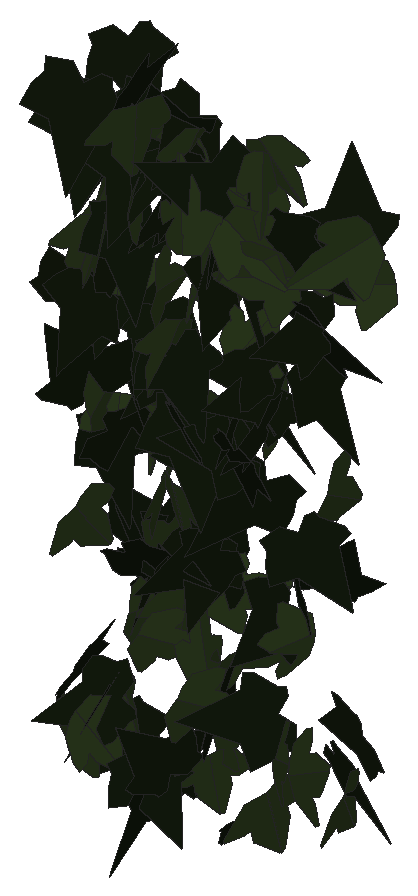
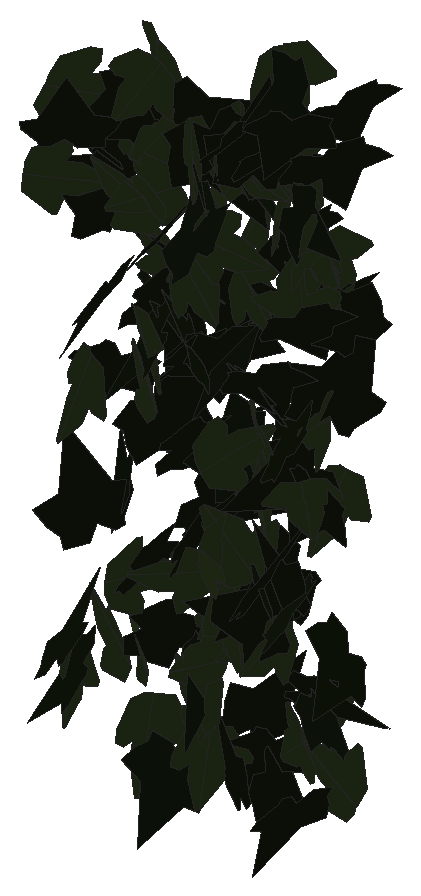
# SketchUp Ruby script. Lengths in inches.
U = 1.inch
M = Sketchup.active_model
def pt(a) = Geom::Point3d.new(a.map { |v| v * U })
def face(e, loops, mat)
  f = e.add_face(loops[0].map { |a| pt(a) })
  loops[1..].each { |l| e.add_face(l.map { |a| pt(a) }).erase! }
  f.material = f.back_material = mat if mat
  f
end
# faces: each face lists its corners as indices into pts; further lists are holes
def faces(e, pts, list, mat = nil) = list.each { |f| face(e, (f[0].is_a?(Array) ? f : [f]).map { |l| l.map { |i| pts[i] } }, mat) }
# xy, xz, yz: faces in a plane at the given z, y or x. An outline is a flat list of corners, or four numbers for a rectangle; further outlines are holes
def ring(l) = l.size == 4 ? [[l[0], l[1]], [l[2], l[1]], [l[2], l[3]], [l[0], l[3]]] : l.each_slice(2).to_a
def flat(e, list, mat, &to3) = list.each { |f| face(e, (f[0].is_a?(Array) ? f : [f]).map { |l| ring(l).map { |u, v| to3.(u, v) } }, mat) }
def xy(e, z, list, mat = nil) = flat(e, list, mat) { |x, y| [x, y, z] }
def xz(e, y, list, mat = nil) = flat(e, list, mat) { |x, z| [x, y, z] }
def yz(e, x, list, mat = nil) = flat(e, list, mat) { |y, z| [x, y, z] }
def lines(e, pts, list) = list.each { |a, b| e.add_line(pt(pts[a]), pt(pts[b])) }
# prism: a flat outline (further loops are holes) pulled along v
def prism(e, loops, v, mat = nil)
  f = face(e, loops, mat); d = Geom::Vector3d.new(v.map { |x| x * U })
  f.pushpull(f.normal.samedirection?(d) ? d.length : -d.length)
end
def box(e, o, s, mat = nil) = prism(e, [[o, [o[0] + s[0], o[1], o[2]], [o[0] + s[0], o[1] + s[1], o[2]], [o[0], o[1] + s[1], o[2]]]], [0, 0, s[2]], mat)
def at(x, y, z, deg = 0) = Geom::Transformation.translation(pt([x, y, z])) * Geom::Transformation.rotation(ORIGIN, Z_AXIS, deg.degrees)
def axes(o, x, y, z) = Geom::Transformation.new([*x, 0, *y, 0, *z, 0, *pt(o).to_a, 1])
def part(name) = M.definitions.add(name)
# library, detail: a bought-in or finely detailed component or shape, given as its bounding box
def library(name, o, s) = part(name).tap { |d| box(d.entities, o, s) }
def detail(e, o, s) = box(e.add_group.entities, o, s)
def put(e, d, t, mat = nil) = e.add_instance(d, t).tap { |i| i.material = mat if mat }
def group(e, t, mat = nil) = e.add_group.tap { |g| g.transformation = t; g.material = mat if mat }.entities
root = M.entities
M.materials.add("efeu1").color = [18, 25, 13]
M.materials.add("efeu2").color = [43, 57, 29]
c1 = part("ivyleaf_10")
p = [[0,0.5,-0.03],[-0.0625,2.02,-0.43],[-0.19,2.01,-0.46],[-0.54,1.05,-0.29],[-0.52,0.625,-0.18],[-0.83,0.76,-0.28],
  [-1.16,0.64,-0.33],[-1.15,0.33,-0.24],[-0.77,-0.39,0.02],[-0.3,-0.51,0.16],[0.04,-0.48,0.23],[-0.02,2.01,-0.4375],
  [-0.06,2.01,-0.43],[0.04,-0.49,0.23],[0.67,-0.49,0.14],[1.38,0.36,-0.2],[1.375,0.51,-0.24],[0.81,0.65,-0.19],
  [0.62,0.59,-0.15],[0.6,1.09,-0.28],[0.5,1.23,-0.31]]
faces(c1.entities,p,[[0,1,2,3,4,5,6,7,8,9,10],[11,12,0,13,14,15,16,17,18,19,20]],"efeu2")
c2 = part("ivyleaf_9")
p = [[1.54,2.16,1.25],[1.36,2.04,1.19],[-0.21,0.99,0.68],[-0.71,1.11,0.82],[-0.85,0.86,0.67],[-0.8,0.17,0.21],
  [-0.9,-0.01,0.1],[-0.67,-0.16,-0.02],[-0.08,-0.08,-0.05],[-0.03,-0.6,-0.4],[0.65,-0.88,-0.66],[0.83,-0.6,-0.49],
  [1.29,-0.42,-0.43],[1.8125,-0.07,-0.26],[1.21,0.44,0.15]]
faces(c2.entities,p,[[0,1,2,3,4,5,6,7,8,9,10,11,12,13,14]],"efeu1")
put(root,c1,axes([551.7,129.9,193.51],[-0.22343,-0.76212,-0.59809],[0.1909,0.56712,-0.79397],[0.94979,-0.29327,0.01889]))
put(root,c2,axes([557.02,130.01,197.18],[0.67195,0.09743,-0.58653],[-0.58638,-0.03779,-0.67805],[-0.09833,0.89112,0.03537]))
put(root,c2,axes([551.27,130.98,199.67],[-0.22153,-0.82284,0.36012],[-0.09205,-0.34816,-0.85214],[0.89346,-0.23989,0.0015]))
put(root,c1,axes([553.25,130.34,206.24],[-0.39364,-0.98437,-0.06429],[0.02505,0.05922,-1.06016],[0.98615,-0.39443,0.00127]))
put(root,c2,axes([550.91,130.95,206.06],[-0.26139,-1.01728,-0.03229],[0.00866,0.03112,-1.05033],[1.01776,-0.26153,0.00064]))
put(root,c1,axes([551.83,130,186.88],[0.07493,0.79738,0.51971],[0.03298,0.51883,-0.80078],[-0.95122,0.0808,0.01317]))
put(root,c2,axes([553.98,130.88,185.74],[0.22147,0.16104,0.80389],[-0.69624,-0.40278,0.27249],[0.43293,-0.73011,0.02699]))
put(root,c2,axes([559.02,130.34,195.12],[-0.08835,-0.46455,-0.74307],[0.27342,0.69494,-0.46697],[0.83258,-0.27751,0.0745]))
put(root,c2,axes([557.65,130.48,197.96],[-0.64583,0.58215,-0.09351],[0.06994,-0.06207,-0.86948],[-0.58545,-0.64961,-0.00072]))
put(root,c2,axes([554.7,130.26,197.55],[0.90407,-0.29541,-0.45534],[-0.41902,0.18244,-0.95031],[0.34501,0.99569,0.03903]))
put(root,c1,axes([554.12,130.89,199.51],[-0.01362,-0.86994,0.34595],[0.05119,-0.34616,-0.86845],[0.9348,0.00628,0.0526]))
put(root,c2,axes([555.11,130.9,197.27],[-0.42388,-0.91668,-0.39818],[0.17401,0.35821,-1.00992],[0.98416,-0.45816,0.00707]))
put(root,c2,axes([552.19,130.91,187.42],[-0.74149,-0.04215,0.44705],[-0.44726,-0.00721,-0.74252],[0.03982,-0.8658,-0.01558]))
put(root,c1,axes([554.85,130.5,203.06],[1.00737,-0.17015,0.32042],[-0.31494,0.05924,1.02162],[-0.18007,-1.05544,0.00569]))
put(root,c1,axes([556.63,130.51,203.66],[0.54869,0.18477,0.81134],[0.74743,0.3177,-0.57783],[-0.36572,0.9265,0.03634]))
put(root,c2,axes([559.39,130.69,201.47],[-0.77674,0.32028,0.27419],[-0.25521,0.10031,-0.84017],[-0.3356,-0.81758,0.00433]))
put(root,c2,axes([554.34,130.76,199.15],[-0.34514,-0.49854,-0.67397],[0.48534,0.47546,-0.60023],[0.68353,-0.58932,0.08589]))
put(root,c2,axes([556.11,131.41,196.45],[0.02498,-0.78714,-0.50493],[0.01742,-0.50463,0.78754],[-0.93501,-0.03043,0.00118]))
put(root,c1,axes([557.09,130.94,205.66],[0.78124,-0.3259,0.37248],[0.35968,-0.10427,-0.84561],[0.33998,0.85919,0.03867]))
put(root,c2,axes([551.44,129.99,188.44],[0.08878,0.71867,0.61151],[0.06846,0.60768,-0.72412],[-0.94114,0.112,0.00501]))
put(root,c1,axes([557.88,130.78,202.625],[0.30428,0.05979,-0.98206],[-0.98175,0.08596,-0.29895],[0.06462,1.02451,0.08239]))
put(root,c1,axes([551.5,130.85,201.88],[0.72615,-0.72293,-0.12259],[-0.07186,0.10154,-1.02444],[0.72972,0.72939,0.02111]))
put(root,c2,axes([551.02,131.18,196.66],[0.50959,0.22223,0.84296],[-0.76823,-0.34706,0.55591],[0.41207,-0.92185,-0.00607]))
put(root,c2,axes([553.09,131.34,184.76],[-0.31411,0.29431,-0.81585],[0.5311,-0.62073,-0.4284],[-0.68569,-0.61561,0.04192]))
put(root,c1,axes([554.15,130.29,201.26],[0.06734,-0.27016,-0.88247],[-0.02663,0.88387,-0.27262],[0.92251,0.04524,0.05654]))
put(root,c2,axes([551.68,131.1,187.39],[-0.52529,0.5187,-0.44741],[0.29735,-0.33527,-0.73779],[-0.6171,-0.60308,0.02535]))
put(root,c2,axes([555.11,131.58,192.72],[-0.15654,-0.10174,-0.85456],[0.0375,-0.86856,0.09653],[-0.85977,-0.01936,0.1598]))
put(root,c1,axes([551.05,131.25,201.6],[-0.20787,-0.89241,0.2302],[0.00276,-0.23659,-0.91467],[0.92162,-0.20057,0.05466]))
put(root,c2,axes([553.11,131,185.56],[-0.21555,-0.50578,-0.64108],[0.25947,0.58625,-0.54976],[0.77425,-0.33728,0.00577]))
put(root,c2,axes([555.98,131.38,203.95],[-0.32139,0.10096,1.00271],[-1.00772,-0.04337,-0.31863],[0.0107,-1.05206,0.10936]))
put(root,c2,axes([557.25,131.05,199.4],[-0.64746,0.34529,0.47022],[-0.43417,0.18399,-0.73293],[-0.38965,-0.77876,0.03533]))
put(root,c1,axes([558.09,131.5,186.86],[0.3952,-0.30601,-0.93342],[0.70563,-0.61151,0.49924],[-0.68338,-0.80839,-0.02431]))
put(root,c2,axes([555.79,130.87,196.5],[-0.30539,0.7564,0.28371],[0.02381,-0.29475,0.81146],[0.80751,0.29476,0.08337]))
put(root,c1,axes([557.22,131.63,187.02],[0.17803,-0.28673,-0.85954],[0.48288,-0.71119,0.33726],[-0.76671,-0.51449,0.01282]))
put(root,c2,axes([557,131.87,198.33],[0.11039,-0.57035,-0.66871],[0.12538,-0.65685,0.58094],[-0.86992,-0.16705,-0.00113]))
put(root,c1,axes([554.93,130.61,188.43],[-0.29325,-0.4429,-0.82357],[0.44216,0.69486,-0.53112],[0.82397,-0.53051,-0.0081]))
put(root,c2,axes([550.4,131,199.26],[-0.19451,-0.02702,0.88712],[0.87275,-0.17085,0.18616],[0.16127,0.89198,0.06253]))
put(root,c1,axes([559.89,131.74,203.9],[0.30916,0.3457,-0.98261],[-0.66001,-0.72796,-0.46376],[-0.80587,0.72882,0.00286]))
put(root,c1,axes([554.79,131.32,201.75],[0.59137,-0.71726,0.00658],[0.00422,-0.00505,-0.92962],[0.71728,0.59139,0.00004]))
put(root,c1,axes([554.2,131.01,194.48],[-0.77999,0.3281,0.11887],[-0.11176,0.04089,-0.84617],[-0.33059,-0.78794,0.00559]))
put(root,c2,axes([552.04,131.5,202.01],[-0.02236,-0.96485,-0.17622],[0.01726,0.17585,-0.96502],[0.98066,-0.0251,0.01297]))
put(root,c2,axes([558.46,131.46,200.82],[0.52594,-0.45764,0.81289],[0.65675,-0.48107,-0.69575],[0.66249,0.84022,0.04439]))
put(root,c2,axes([557.6,130.98,203.78],[0.011,-0.07092,-0.97432],[0.64691,0.73065,-0.04588],[0.73201,-0.64465,0.05518]))
put(root,c2,axes([552.42,131.75,204.1],[-0.56426,-0.73088,-0.0575],[0.03558,0.04517,-0.92335],[0.73227,-0.56538,0.00056]))
put(root,c2,axes([556.87,131.85,188.14],[-0.21313,-0.42032,-0.7923],[-0.28031,-0.74235,0.46923],[-0.85196,0.3494,0.04382]))
put(root,c2,axes([554.9,131.96,200.91],[-0.00342,-0.72917,0.49874],[0.02632,-0.49861,-0.7288],[0.88303,0.01204,0.02365]))
put(root,c2,axes([556.53,131.83,195.25],[-0.00102,0.24337,-0.98585],[-0.04123,-0.98505,-0.24313],[-1.01461,0.03979,0.01087]))
put(root,c1,axes([550.18,131.49,185.26],[-0.42958,-0.05843,0.8945],[0.89489,0.02971,0.43171],[-0.05211,0.99186,0.03976]))
put(root,c2,axes([553.9,131.45,203.59],[-0.76919,0.56427,-0.18567],[0.14566,-0.11532,-0.95394],[-0.5759,-0.78283,0.0067]))
put(root,c1,axes([556.625,131.16,203.02],[-0.39177,-0.68563,-0.50952],[0.25744,0.43972,-0.78966],[0.81451,-0.46877,0.00451]))
put(root,c2,axes([550.625,131.95,204.97],[-0.4664,-0.9382,-0.16477],[0.05852,0.15489,-1.04761],[0.95076,-0.46977,-0.01634]))
put(root,c2,axes([554.52,132.11,192.47],[-0.16655,-0.8812,0.23032],[-0.03899,-0.22703,-0.89679],[0.90997,-0.17101,0.00373]))
put(root,c1,axes([556.125,131.42,199.42],[0.7912,-0.07752,-0.50345],[0.50679,0.02601,0.79243],[-0.05137,-0.93743,0.06362]))
put(root,c2,axes([554.625,131.79,204.27],[0.24152,0.51878,-0.876],[-0.33235,-0.81081,-0.57181],[-0.96232,0.41022,-0.02237]))
put(root,c1,axes([553.1875,131.72,194.25],[0.38823,-0.91558,-0.07321],[-0.0254,0.06875,-0.99448],[0.91815,0.38905,0.00345]))
put(root,c1,axes([554.79,131.39,189.1875],[-0.16395,0.95139,-0.28525],[-0.08304,0.27497,0.96483],[0.98976,0.18067,0.0337]))
put(root,c2,axes([557.44,132.3125,192.03],[0.02364,-0.21488,0.90008],[0.17762,-0.88258,-0.21537],[0.90816,0.17821,0.01869]))
put(root,c1,axes([551.23,131.1,196.18],[-0.0227,0.24114,-0.87397],[-0.00132,0.87423,0.24125],[0.90662,0.00731,-0.02153]))
put(root,c1,axes([552.09,132.02,204.82],[-0.60582,-0.47256,0.57757],[-0.4577,-0.35229,-0.76832],[0.58941,-0.75928,-0.00298]))
put(root,c1,axes([552.98,131.37,189.4375],[-0.29184,-0.32166,-0.72533],[0.4916,0.53333,-0.43431],[0.62282,-0.57169,0.00294]))
put(root,c1,axes([552.55,131.21,202.63],[-0.0849,0.22237,0.91702],[-0.588,0.70764,-0.22604],[-0.738,-0.58939,0.0746]))
put(root,c1,axes([556.8,131.7,185.44],[-0.29923,-1.00001,-0.37227],[0.08673,0.36256,-1.04363],[1.06352,-0.31093,-0.01964]))
put(root,c1,axes([556.4,132.28,203.34],[-0.02746,0.65443,0.5911],[-0.0218,-0.59171,0.65409],[0.88159,0.00575,0.03459]))
put(root,c2,axes([552.18,131.08,205.77],[0.17953,0.36068,0.93092],[0.27147,0.89258,-0.39818],[-0.96073,0.31961,0.06145]))
put(root,c2,axes([552.74,132.24,191.68],[-0.59058,0.21078,-0.58776],[0.52833,-0.2625,-0.625],[-0.33279,-0.79078,0.05081]))
put(root,c2,axes([554.83,132.29,203.46],[-0.46981,0.10038,-0.74397],[0.70712,-0.23553,-0.47832],[-0.25208,-0.84778,0.0448]))
put(root,c2,axes([551.22,132.4,199.97],[-0.49425,-0.77119,-0.08333],[0.05339,0.06475,-0.91592],[0.77384,-0.49703,0.00997]))
put(root,c1,axes([551.52,131.79,200.01],[0.80082,0.51694,-0.08392],[0.06066,0.06074,0.953],[0.52018,-0.80291,0.01806]))
put(root,c1,axes([552.56,132.34,196.1],[0.71955,-0.49984,0.33483],[0.25606,-0.21791,-0.87559],[0.54441,0.76313,-0.03071]))
put(root,c2,axes([552.05,131.6,191.55],[0.91361,0.31637,0.12177],[0.11592,0.03738,-0.96683],[-0.31856,0.92093,-0.00259]))
put(root,c1,axes([551.1,132.35,186.78],[0.48679,-0.18862,0.73526],[0.71458,-0.18078,-0.51947],[0.25606,0.86307,0.05188]))
put(root,c1,axes([559.39,131.76,186.37],[0.07782,-0.75674,-0.58203],[-0.06318,0.5786,-0.76073],[0.95259,0.1002,-0.00291]))
put(root,c1,axes([553.43,132.51,204.51],[0.07132,-0.82464,0.38496],[0.08731,-0.37816,-0.82625],[0.90588,0.10137,0.04933]))
put(root,c2,axes([550.76,132.26,194.73],[-0.48236,-0.19036,-0.79523],[0.71925,0.34043,-0.51776],[0.38897,-0.86554,-0.02875]))
put(root,c1,axes([554.52,132.35,186.42],[-0.61619,0.08013,0.74335],[0.7336,-0.12115,0.62117],[0.14433,0.95791,0.01638]))
put(root,c1,axes([556.92,132.87,190.07],[-0.03009,-0.04578,0.92637],[-0.03309,-0.92622,-0.04684],[0.92691,-0.03455,0.0284]))
put(root,c2,axes([556.37,132.94,190.65],[-0.22169,-0.61773,0.64797],[-0.22237,-0.60862,-0.6563],[0.86719,-0.31399,-0.00265]))
put(root,c1,axes([556.55,132.1,205.56],[-0.79049,0.02593,-0.4214],[0.4209,-0.02151,-0.79089],[-0.033,-0.89554,0.00679]))
put(root,c2,axes([554.99,132.92,194.85],[-0.04449,-0.80674,-0.57929],[-0.0385,-0.57804,0.80795],[-0.99243,0.05859,-0.00537]))
put(root,c2,axes([554.79,132.94,191.64],[-0.21281,-0.20613,0.86124],[-0.29606,-0.81823,-0.26899],[0.83461,-0.34281,0.12418]))
put(root,c2,axes([552,132.76,205.06],[-0.22546,-0.87355,0.10052],[-0.02723,-0.09678,-0.90217],[0.87889,-0.22709,-0.00217]))
put(root,c1,axes([554.46,132.17,185.59],[-0.5392,-0.71453,-0.14688],[0.10101,0.10775,-0.89501],[0.72244,-0.54836,0.01551]))
put(root,c2,axes([553.07,132.39,195.16],[0.74777,-0.43328,0.56399],[0.46937,-0.31418,-0.86369],[0.53433,0.88235,-0.03059]))
put(root,c1,axes([553.37,132.33,190.41],[-0.44049,-0.84952,0.01286],[-0.00085,-0.01404,-0.95691],[0.84961,-0.44045,0.00571]))
put(root,c2,axes([555.65,132.78,201.23],[0.12081,-0.88095,0.22752],[0.05536,-0.22197,-0.88887],[0.90817,0.13072,0.02392]))
put(root,c2,axes([556.15,132.23,197.73],[0.77788,-0.44693,-0.23945],[-0.19429,0.1423,-0.89676],[0.46833,0.80136,0.02569]))
put(root,c2,axes([552.95,132.56,197.625],[-0.84366,0.13671,-0.09247],[0.09159,-0.01285,-0.85466],[-0.1373,-0.84861,-0.00196]))
put(root,c2,axes([551.27,132.56,191.26],[-0.10391,0.16615,0.82796],[0.5004,-0.65986,0.19522],[0.68024,0.51079,-0.01713]))
put(root,c1,axes([554.92,132.25,204.33],[0.20001,-0.8185,-0.31435],[-0.05147,0.31091,-0.84229],[0.87528,0.20532,0.0223]))
put(root,c2,axes([552.53,132.66,204.25],[0.71258,0.16441,0.50191],[-0.48551,-0.12791,0.73119],[0.20792,-0.86216,-0.01277]))
put(root,c1,axes([554.64,132.79,200.47],[-0.00819,-0.90582,0.37714],[0.00716,-0.3772,-0.9058],[0.98117,-0.00481,0.00976]))
put(root,c2,axes([553.01,132.66,184.8],[-0.15469,0.27045,0.80369],[0.3186,-0.73856,0.30986],[0.78585,0.35267,0.03258]))
put(root,c2,axes([553.2,133.11,204.98],[-0.26417,-0.75655,0.4145],[-0.15179,-0.38598,-0.80122],[0.8492,-0.30434,-0.01427]))
put(root,c2,axes([551.25,131.8,195.02],[0.01238,0.26448,-0.88],[0.08001,0.87643,0.26454],[0.9154,-0.08018,-0.01122]))
put(root,c1,axes([553.29,132.62,204.11],[0.3938,0.03391,-0.76463],[-0.76308,-0.04923,-0.39519],[-0.0593,0.85867,0.00754]))
put(root,c1,axes([556.37,132.49,201.59],[0.54393,-0.13561,-0.83686],[0.83287,-0.10017,0.55757],[-0.15829,-0.99306,0.05804]))
put(root,c1,axes([550.49,133.04,202.64],[-0.00374,0.38664,-0.74683],[0.00493,-0.74681,-0.38666],[-0.84096,-0.0061,0.00105]))
put(root,c1,axes([552.97,132.43,191.82],[-0.51918,-0.63949,0.49513],[0.3832,0.32363,0.8198],[-0.71223,0.64028,0.08015]))
put(root,c1,axes([554.55,131.86,187.9375],[0.10808,-0.30144,0.9377],[-0.23626,0.90785,0.31907],[-0.9562,-0.25839,0.02715]))
put(root,c2,axes([554.92,131.87,187.75],[-0.19206,0.11433,-1.0557],[-0.87815,0.58607,0.22323],[0.59701,0.89884,-0.01127]))
put(root,c2,axes([550.85,132.91,203.72],[-0.42502,0.32031,-0.6481],[0.41192,-0.51052,-0.52245],[-0.59409,-0.58313,0.1014]))
put(root,c2,axes([557.73,132.49,198.75],[0.4906,-0.7094,-0.43293],[-0.21637,0.37637,-0.86191],[0.80241,0.53522,0.03228]))
put(root,c1,axes([555.85,132.27,202.33],[0.36671,0.14062,0.84622],[0.69743,0.48695,-0.38315],[-0.49945,0.78323,0.08629]))
put(root,c1,axes([556.49,132.51,198.06],[0.69504,-0.55146,-0.36174],[-0.24318,0.27423,-0.88527],[0.61305,0.73399,0.05897]))
put(root,c2,axes([550.98,133.17,196.2],[0.13705,-0.60882,0.63453],[0.24755,-0.58951,-0.61909],[0.84381,0.27183,0.07857]))
put(root,c1,axes([551.98,132.02,189.67],[-0.04878,-0.21112,-0.88256],[0.20789,0.85773,-0.21667],[0.88333,-0.21352,0.00226]))
put(root,c2,axes([551.79,132.52,190.39],[0.51458,-0.08083,0.79105],[0.78008,-0.13141,-0.52087],[0.15421,0.9345,-0.00482]))
put(root,c1,axes([558.71,132.09,195.58],[-0.00176,-0.61601,-0.92274],[-0.00831,0.92272,-0.61598],[1.10944,0.00593,-0.00608]))
put(root,c2,axes([555.68,132.125,184.41],[0.26664,0.81799,0.29214],[0.08093,0.28087,-0.8603],[-0.86481,0.27849,0.00956]))
put(root,c2,axes([558.43,132.73,186.875],[0.75966,-0.52793,-0.14012],[-0.11444,0.08087,-0.92509],[0.53409,0.76823,0.00109]))
put(root,c1,axes([550.62,132.85,195.05],[0.64529,0.5381,-0.09299],[-0.07188,-0.059,-0.84021],[-0.54132,0.64928,0.00072]))
put(root,c2,axes([558.66,133.41,187.41],[0.58601,-0.6927,-0.2414],[0.1548,-0.18524,0.90732],[-0.71704,-0.60611,-0.0014]))
put(root,c1,axes([559.46,133.125,201.9375],[0.11294,0.00293,-0.93995],[-0.89523,-0.28821,-0.10846],[-0.28648,0.90177,-0.03161]))
put(root,c2,axes([552.3,133.23,191.13],[0.00229,-0.95208,0.10893],[0.05983,0.10886,0.95021],[-0.95642,0.00453,0.0597]))
put(root,c1,axes([554.67,132.4375,190.91],[0.10413,-0.07878,-0.89708],[0.74612,0.51321,0.04154],[0.50425,-0.74311,0.12379]))
put(root,c1,axes([555.92,132.9375,196.1],[0.533,-0.74913,-0.00724],[0.00826,-0.00301,0.91938],[-0.74912,-0.53304,0.00499]))
put(root,c2,axes([551.82,133.35,198.44],[-0.55708,-0.68406,-0.15095],[0.10227,0.11137,-0.88216],[0.69302,-0.56632,0.00884]))
put(root,c1,axes([553.77,132.98,201.82],[0.17806,0.10545,-0.89522],[-0.89733,0.10744,-0.16582],[0.08565,0.90641,0.1238]))
put(root,c1,axes([553.18,133.48,195.35],[-0.32087,-0.20047,-0.81756],[-0.61608,-0.54029,0.37428],[-0.57362,0.69243,0.05535]))
put(root,c2,axes([550.68,133.33,191.44],[0.41557,-0.76758,0.18436],[0.10147,-0.15468,-0.87272],[0.78286,0.42751,0.01525]))
put(root,c2,axes([557.62,133.14,191.87],[0.8404,0.36729,0.12652],[-0.12517,-0.02944,0.91687],[0.36775,-0.84936,0.02294]))
put(root,c2,axes([558.86,132.84,203.17],[-0.78197,-0.30162,0.41554],[0.39753,0.12353,0.83775],[-0.32498,0.87686,0.02491]))
put(root,c1,axes([553.31,133.59,192.46],[0.26069,-0.57064,0.65422],[0.29686,-0.5833,-0.62707],[0.81579,0.39461,0.01913]))
put(root,c2,axes([550.81,132.95,185.27],[0.1729,-0.71736,-0.57502],[-0.09718,0.56756,-0.73727],[0.91422,0.196,0.03038]))
put(root,c2,axes([553.72,133.6,201.79],[0.823,-0.38854,-0.39815],[0.36348,-0.16267,0.91007],[-0.42115,-0.89966,0.0074]))
put(root,c2,axes([550.81,133.13,206.52],[-0.24135,-0.6222,-0.57073],[0.25197,0.51346,-0.66632],[0.80584,-0.3469,0.03741]))
